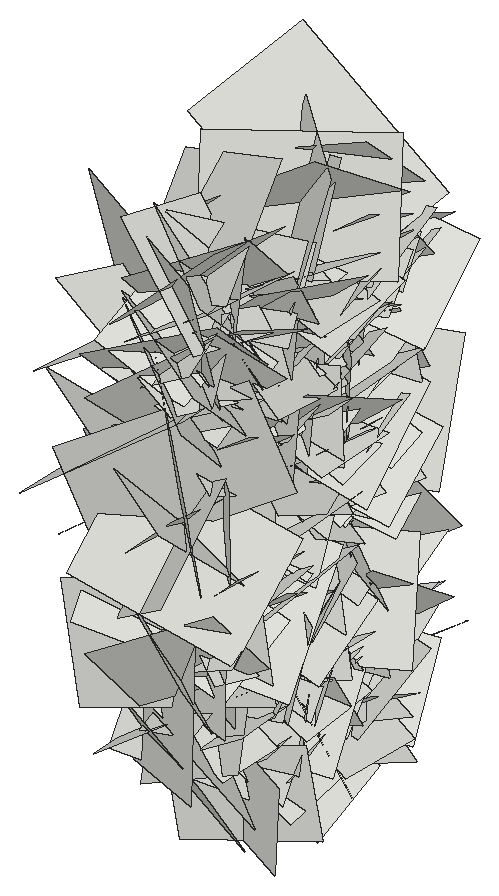
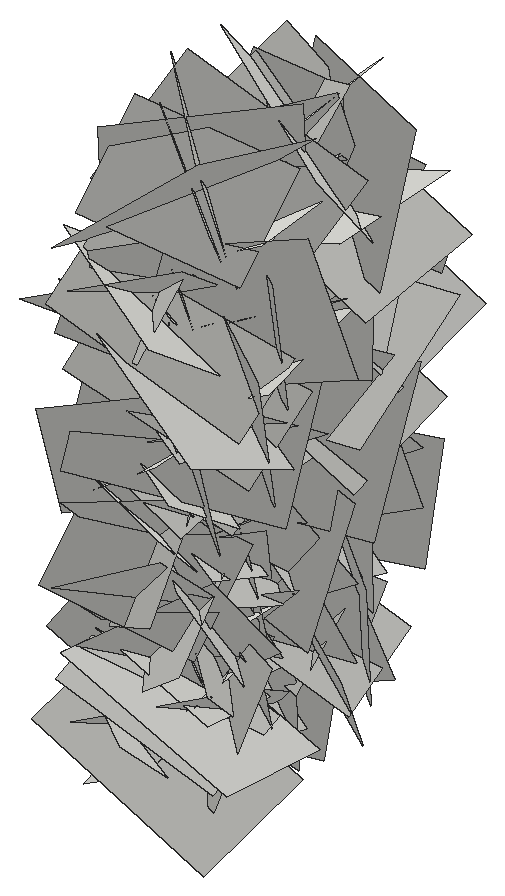
# SketchUp Ruby script. Lengths in inches.
U = 1.inch
M = Sketchup.active_model
def pt(a) = Geom::Point3d.new(a.map { |v| v * U })
def face(e, loops, mat)
  f = e.add_face(loops[0].map { |a| pt(a) })
  loops[1..].each { |l| e.add_face(l.map { |a| pt(a) }).erase! }
  f.material = f.back_material = mat if mat
  f
end
# faces: each face lists its corners as indices into pts; further lists are holes
def faces(e, pts, list, mat = nil) = list.each { |f| face(e, (f[0].is_a?(Array) ? f : [f]).map { |l| l.map { |i| pts[i] } }, mat) }
# xy, xz, yz: faces in a plane at the given z, y or x. An outline is a flat list of corners, or four numbers for a rectangle; further outlines are holes
def ring(l) = l.size == 4 ? [[l[0], l[1]], [l[2], l[1]], [l[2], l[3]], [l[0], l[3]]] : l.each_slice(2).to_a
def flat(e, list, mat, &to3) = list.each { |f| face(e, (f[0].is_a?(Array) ? f : [f]).map { |l| ring(l).map { |u, v| to3.(u, v) } }, mat) }
def xy(e, z, list, mat = nil) = flat(e, list, mat) { |x, y| [x, y, z] }
def xz(e, y, list, mat = nil) = flat(e, list, mat) { |x, z| [x, y, z] }
def yz(e, x, list, mat = nil) = flat(e, list, mat) { |y, z| [x, y, z] }
def lines(e, pts, list) = list.each { |a, b| e.add_line(pt(pts[a]), pt(pts[b])) }
# prism: a flat outline (further loops are holes) pulled along v
def prism(e, loops, v, mat = nil)
  f = face(e, loops, mat); d = Geom::Vector3d.new(v.map { |x| x * U })
  f.pushpull(f.normal.samedirection?(d) ? d.length : -d.length)
end
def box(e, o, s, mat = nil) = prism(e, [[o, [o[0] + s[0], o[1], o[2]], [o[0] + s[0], o[1] + s[1], o[2]], [o[0], o[1] + s[1], o[2]]]], [0, 0, s[2]], mat)
def at(x, y, z, deg = 0) = Geom::Transformation.translation(pt([x, y, z])) * Geom::Transformation.rotation(ORIGIN, Z_AXIS, deg.degrees)
def axes(o, x, y, z) = Geom::Transformation.new([*x, 0, *y, 0, *z, 0, *pt(o).to_a, 1])
def part(name) = M.definitions.add(name)
# library, detail: a bought-in or finely detailed component or shape, given as its bounding box
def library(name, o, s) = part(name).tap { |d| box(d.entities, o, s) }
def detail(e, o, s) = box(e.add_group.entities, o, s)
def put(e, d, t, mat = nil) = e.add_instance(d, t).tap { |i| i.material = mat if mat }
def group(e, t, mat = nil) = e.add_group.tap { |g| g.transformation = t; g.material = mat if mat }.entities
root = M.entities
c1 = part("Component\#6")
p = [[0.01,0,0],[0,3.24,4.54],[4.32,3.24,4.54],[4.33,0,0]]
faces(c1.entities,p,[[0,1,2,3]])
put(root,c1,axes([18.5,202.95,19.72],[-0.19445,-0.3512,-1.29554],[-0.25274,-1.27827,0.38028],[-1.40021,0.2795,0.11127]))
put(root,c1,axes([18.5,194.4,9.86],[-0.11876,-1.04596,0.91618],[-0.1474,0.92297,1.03671],[-1.46651,-0.00807,-0.1784]))
put(root,c1,axes([18.5,199.09,4.9],[-0.11121,1.25407,0.182],[-0.25083,0.16003,-1.23904],[-1.31962,-0.1361,0.22018]))
put(root,c1,axes([18.5,192.59,17.15],[-0.08597,-0.32374,1.28455],[-0.18245,1.27862,0.31138],[-1.3923,-0.14756,-0.12012]))
put(root,c1,axes([18.5,193.34,3.5],[-0.3285,0.68164,0.95344],[-0.04901,0.97833,-0.71446],[-1.2414,-0.219,-0.22409]))
put(root,c1,axes([18.5,197.84,15.77],[-0.08558,0.66637,-1.22765],[-0.01617,-1.23004,-0.66667],[-1.48057,-0.02508,0.07824]))
put(root,c1,axes([18.5,196.95,13.22],[-0.12152,0.35472,1.26895],[-0.01769,1.27325,-0.35743],[-1.39654,-0.047,-0.10589]))
put(root,c1,axes([18.5,198.6875,16.83],[-0.02201,1.26014,0.56955],[-0.0456,0.56875,-1.25994],[-1.46513,-0.03663,0.03065]))
put(root,c1,axes([18.5,191.67,21.5],[-0.0579,1.33618,-0.15223],[-0.05318,-0.15428,-1.33612],[-1.42453,-0.04855,0.05606]))
put(root,c1,axes([18.5,196.26,4.8],[-0.10051,-0.43998,1.12809],[-0.21352,1.12151,0.42048],[-1.26562,-0.15427,-0.16053]))
put(root,c1,axes([18.5,201.79,17.38],[-0.19939,0.73728,-1.06028],[0.09629,-1.06126,-0.75408],[-1.36551,-0.18249,0.10164]))
put(root,c1,axes([18.5,195.52,16.87],[-0.17814,-1.09516,0.21581],[-0.19304,0.24222,1.08736],[-1.16734,0.12707,-0.21275]))
put(root,c1,axes([18.5,190.86,3.39],[-0.21383,0.32739,1.20741],[0.09698,1.22359,-0.31649],[-1.32251,0.03679,-0.21843]))
put(root,c1,axes([18.5,190.45,18.05],[-0.16537,1.24759,-0.14593],[0.05265,-0.14081,-1.25691],[-1.33042,-0.16065,-0.0316]))
put(root,c1,axes([18.5,200.21,21.54],[-0.14018,1.21556,-0.55877],[0.14242,-0.54659,-1.22085],[-1.41094,-0.17594,-0.06772]))
put(root,c1,axes([18.5,192.73,15.73],[-0.12897,1.2724,-0.23633],[0.08155,-0.22984,-1.27707],[-1.36939,-0.13352,-0.05379]))
put(root,c1,axes([18.5,200.25,4.79],[-0.06637,1.27776,-0.24675],[0.01199,-0.2465,-1.2793],[-1.3794,-0.06362,0.00075]))
put(root,c1,axes([18.5,199.38,-0.0625],[-0.15183,-0.50198,1.07326],[-0.00307,1.08122,0.50532],[-1.25594,0.05804,-0.13098]))
put(root,c1,axes([18.5,192.7,21.39],[-0.08893,0.79245,0.9015],[-0.06254,0.89988,-0.79652],[-1.27076,-0.09974,-0.02389]))
put(root,c1,axes([18.5,194.09,6.34],[-0.25898,1.07168,-0.21064],[0.01285,-0.21318,-1.09862],[-1.15764,-0.24212,0.03493]))
put(root,c1,axes([18.5,200.7,5.85],[-0.20906,1.0682,-0.14016],[-0.07965,-0.15578,-1.08152],[-1.13921,-0.18514,0.10133]))
put(root,c1,axes([18.5,198.85,12.57],[-0.15345,0.48368,1.12599],[0.09378,1.13498,-0.47617],[-1.29562,0.02486,-0.16783]))
put(root,c1,axes([18.5,195.93,15.54],[-0.04965,0.25406,1.2028],[-0.02984,1.20314,-0.25523],[-1.30276,-0.03724,-0.03999]))
put(root,c1,axes([18.5,204.42,20.53],[-0.1154,-1.25003,-0.28156],[0.14973,-0.29256,1.24425],[-1.34995,0.07441,0.16208]))
put(root,c1,axes([18.5,199.56,18.73],[-0.07364,1.07871,-0.62029],[0.05176,-0.61841,-1.08091],[-1.31797,-0.08456,-0.00779]))
put(root,c1,axes([18.5,203.04,12.11],[-0.14841,-0.94408,-0.5752],[-0.05434,-0.57362,0.95398],[-1.17058,0.14632,0.02864]))
put(root,c1,axes([18.5,200.375,7.61],[-0.26418,-0.51362,-0.84712],[-0.05211,-0.86603,0.53955],[-1.04881,0.1724,0.18657]))
put(root,c1,axes([18.5,197.84,4.84],[-0.11369,-0.36766,-0.96616],[-0.19069,-0.94989,0.38144],[-1.07906,0.2066,0.03439]))
put(root,c1,axes([18.5,197.86,18.23],[-0.19608,0.2602,-1.0463],[0.01915,-1.06069,-0.26697],[-1.14269,-0.06243,0.17507]))
put(root,c1,axes([18.5,202.25,12.93],[0.19135,-1.27912,0.12446],[-0.2118,0.09622,1.27869],[-1.34571,-0.19703,-0.18355]))
put(root,c1,axes([18.5,198.375,11.05],[0.00636,-0.47599,-1.14741],[0.03555,-1.14695,0.47597],[-1.31628,-0.03327,0.00731]))
put(root,c1,axes([18.5,200.2,14.91],[-0.20407,-0.96139,-0.18597],[-0.07393,-0.17559,0.97991],[-1.03533,0.20204,-0.03331]))
put(root,c1,axes([18.5,196.53,2.03],[-0.14871,0.38131,0.94323],[-0.09041,0.94439,-0.39446],[-1.07463,-0.13222,-0.09734]))
put(root,c1,axes([18.5,192.66,5.0625],[-0.03803,0.06475,1.02957],[-0.25075,1.00223,-0.07127],[-1.06436,-0.23842,-0.02]))
put(root,c1,axes([18.5,199.09,16.39],[-0.13116,-1.14374,0.05938],[0.13174,0.04596,1.1443],[-1.20683,0.12933,0.11846]))
put(root,c1,axes([18.5,200.08,24.34],[-0.03463,0.75517,-0.67877],[-0.20748,-0.67107,-0.73718],[-1.05612,0.10708,0.16708]))
put(root,c1,axes([14.53,199.42,15.6],[-0.03605,-0.49998,-0.38134],[-0.14474,-0.36691,0.49324],[0.65063,-0.10932,0.0886]))
put(root,c1,axes([14.53,199.74,12.37],[-0.13977,-0.41949,-0.41774],[0.0557,-0.43458,0.41982],[0.62506,-0.05508,-0.13082]))
put(root,c1,axes([18.5,197.36,24.8],[0.09794,1.0389,-0.68546],[0.01654,-0.68826,-1.04104],[-1.31923,0.0685,-0.06394]))
put(root,c1,axes([18.5,194.35,10.5],[0.1187,0.07765,-1.12146],[-0.14385,-1.11784,-0.09095],[-1.18288,0.14373,-0.10148]))
put(root,c1,axes([18.5,194.25,1.05],[-0.1707,-0.55728,0.79671],[0.04122,0.80323,0.5697],[-1.02978,0.12452,-0.10926]))
put(root,c1,axes([18.5,205.24,14.9],[0.1168,-0.46047,-1.13614],[0.0362,-1.13913,0.465],[-1.29896,-0.07315,-0.0892]))
put(root,c1,axes([18.5,200.51,5.45],[0.07717,-0.59417,-0.91785],[-0.09928,-0.91989,0.58806],[-1.15472,0.03938,-0.1119]))
put(root,c1,axes([14.53,194.11,10.49],[-0.01019,-0.66626,0.06574],[-0.1187,0.06642,0.65679],[0.69967,0.00157,0.11238]))
put(root,c1,axes([18.5,202.1,18.26],[0.1919,-1.13475,-0.09678],[-0.16378,-0.12156,1.13628],[-1.19604,-0.16542,-0.17113]))
put(root,c1,axes([18.5,198.84,9.75],[0.24721,-0.9594,-0.88495],[0.06038,-0.89063,0.98057],[-1.38221,-0.2105,-0.11544]))
put(root,c1,axes([18.5,198.93,5.125],[-0.08676,0.85287,0.14934],[-0.16568,0.13299,-0.84515],[-0.90272,-0.10637,0.14076]))
put(root,c1,axes([18.5,203.91,5.3125],[-0.18463,-0.58129,-0.78091],[0.13848,-0.80009,0.56643],[-1.02258,-0.00339,0.2177]))
put(root,c1,axes([18.5,195.28,4.79],[-0.03702,0.87634,0.85063],[0.28559,0.83554,-0.84973],[-1.26267,0.16329,-0.21713]))
put(root,c1,axes([18.5,193.71,0.46],[-0.00413,-0.52236,0.7551],[-0.18121,0.74232,0.51263],[-0.95624,-0.13842,-0.10041]))
put(root,c1,axes([18.5,192.44,8.79],[0.05887,1.04295,0.25043],[-0.00297,0.2509,-1.04431],[-1.13694,0.05335,0.0157]))
put(root,c1,axes([14.53,196.1,5.28],[-0.08762,-0.56519,-0.39893],[0.0287,-0.4041,0.56691],[0.73275,-0.05175,-0.06991]))
put(root,c1,axes([14.53,199.53,17.66],[-0.07108,0.22718,0.77768],[-0.14032,0.76678,-0.23541],[0.84726,0.14605,0.02626]))
put(root,c1,axes([14.53,201.03,8.02],[-0.03451,-0.61291,-0.20918],[0.0475,-0.21108,0.61149],[0.68484,-0.01625,-0.05296]))
put(root,c1,axes([14.53,198.53,13.8],[-0.10676,-0.41647,0.70694],[-0.09382,0.7136,0.40779],[0.86465,0.02601,0.13154]))
put(root,c1,axes([18.5,196.19,13.89],[0.03711,0.95345,-0.08325],[-0.1071,-0.07916,-0.94908],[-1.00884,0.04348,0.09769]))
put(root,c1,axes([18.5,197.24,20.32],[-0.11105,0.4932,0.81979],[0.10012,0.82599,-0.48487],[-1.00916,0.02768,-0.13831]))
put(root,c1,axes([14.53,202.56,19.21],[0.06396,-0.26998,-0.58675],[-0.04641,-0.58965,0.26682],[0.68306,-0.01478,0.07307]))
put(root,c1,axes([14.53,199.64,2.06],[-0.21894,0.61345,0.59822],[0.01858,0.61825,-0.62794],[0.90807,0.13525,0.15708]))
put(root,c1,axes([18.5,196.07,8.125],[-0.08332,-0.69698,-0.457],[-0.10667,-0.44773,0.70016],[-0.87699,0.12068,-0.04174]))
put(root,c1,axes([14.53,190.79,19.57],[0.04866,0.55121,0.30162],[0.00575,0.30207,-0.55285],[0.66601,-0.04288,-0.01726]))
put(root,c1,axes([14.53,195.85,11.01],[-0.15114,0.73817,0.19544],[0.07767,0.21113,-0.74396],[0.80568,0.11812,0.10838]))
put(root,c1,axes([18.5,202.76,13.17],[0.11284,-1.03894,-0.17524],[-0.03066,-0.17895,1.04335],[-1.11641,-0.1001,-0.04636]))
put(root,c1,axes([18.5,189.31,11.46],[-0.01967,0.80876,0.77653],[0.21901,0.76581,-0.79265],[-1.16812,0.12996,-0.16169]))
put(root,c1,axes([14.53,193.57,4.75],[0.0218,0.6351,0.02763],[0.03876,0.02642,-0.63443],[0.67273,-0.0221,0.03566]))
put(root,c1,axes([18.5,199.68,18.17],[0.10811,0.81171,0.57509],[-0.11351,0.5837,-0.80488],[-1.04835,0.0205,0.14645]))
put(root,c1,axes([14.53,202.9,8.46],[-0.28421,-0.45126,-0.90988],[-0.10984,-0.92399,0.48879],[1.07096,-0.21452,-0.19133]))
put(root,c1,axes([14.53,193.91,15.9375],[0.03263,0.61645,-0.26034],[-0.02336,-0.25954,-0.61716],[0.70894,-0.03692,-0.00835]))
put(root,c1,axes([14.53,192.26,20.51],[-0.14395,0.6641,-0.62024],[-0.10915,-0.63433,-0.65665],[0.95701,0.02754,-0.16819]))
put(root,c1,axes([14.53,199.23,1.1],[-0.00098,-0.71414,-0.15761],[-0.04174,-0.15733,0.71311],[0.77408,-0.00939,0.03826]))
put(root,c1,axes([14.53,196.5625,6.92],[0.07674,-0.09799,-0.6482],[-0.03176,-0.65195,0.09521],[0.69417,-0.019,0.07601]))
put(root,c1,axes([14.53,198.91,12.75],[-0.15355,-0.10183,1.00426],[-0.21738,0.99636,0.07145],[1.04766,0.19182,0.16201]))
put(root,c1,axes([14.53,195.68,15.75],[0.06715,-0.51242,0.33521],[0.05381,0.34023,0.51051],[0.64683,0.02489,-0.07727]))
put(root,c1,axes([14.53,200.4375,8.06],[-0.17377,0.75884,-0.49804],[-0.05898,-0.51355,-0.76415],[0.96033,0.10576,-0.13705]))
put(root,c1,axes([14.53,199.6875,17.84],[0.07891,0.44569,0.39814],[0.07493,0.39183,-0.45185],[0.62903,-0.10259,0.00388]))
put(root,c1,axes([14.53,200.03,9.27],[-0.00412,-0.60297,0.30435],[0.07057,0.30253,0.60022],[0.71247,-0.03345,-0.05769]))
put(root,c1,axes([14.53,192.95,10.8],[0.02962,0.02518,0.78508],[-0.12702,0.77652,-0.02064],[0.82287,0.11896,-0.03145]))
put(root,c1,axes([18.5,199.37,10.67],[0.09558,-1.01864,0.46326],[0.13943,0.47118,1.01047],[-1.17795,-0.02688,0.1572]))
put(root,c1,axes([14.53,198.38,4.95],[-0.02223,0.32868,-0.55446],[0.17267,-0.53404,-0.32274],[0.66105,0.15055,0.06565]))
put(root,c1,axes([14.53,192.04,10.01],[-0.12172,0.5206,-0.6372],[0.01939,-0.6416,-0.52749],[0.87198,0.08694,-0.07722]))
put(root,c1,axes([14.53,202.51,19.98],[0.06792,0.48446,-0.5602],[-0.10116,-0.55221,-0.48846],[0.77852,-0.11402,-0.01459]))
put(root,c1,axes([18.5,195.86,16.68],[-0.06531,-0.43873,0.684],[-0.07025,0.68639,0.43429],[-0.8585,-0.02279,-0.08757]))
put(root,c1,axes([14.53,202.74,-0.14],[0.03158,-0.64507,0.25861],[0.01592,0.25938,0.64528],[0.73651,0.02205,-0.02503]))
put(root,c1,axes([18.5,192.22,20.81],[-0.00161,0.62306,-0.59539],[-0.0785,-0.59329,-0.62067],[-0.91013,0.05007,0.05459]))
put(root,c1,axes([14.53,197.35,3.52],[0.03443,0.41092,0.66217],[-0.08038,0.66126,-0.40665],[0.82215,0.04744,-0.06748]))
put(root,c1,axes([14.53,195.99,4.23],[-0.18601,0.0566,0.88651],[0.05201,0.90288,-0.04793],[0.94017,-0.03875,0.17804]))
put(root,c1,axes([18.5,198.67,11.97],[0.07539,0.76068,0.50866],[-0.0723,0.51318,-0.75791],[-0.96729,0.02092,0.0963]))
put(root,c1,axes([14.53,195.9375,9.16],[0.07841,0.69576,-0.29748],[-0.09095,-0.28926,-0.69787],[0.79692,-0.10147,-0.05038]))
put(root,c1,axes([18.5,195.4375,18.11],[-0.16874,-0.51977,-0.57708],[0.05885,-0.59519,0.52076],[-0.82114,0.06415,0.15591]))
put(root,c1,axes([18.5,196.17,12.88],[0.06274,0.02618,0.84664],[-0.15393,0.83645,-0.01571],[-0.88457,-0.1437,0.06278]))
put(root,c1,axes([18.5,193.46,10.77],[-0.10152,0.90556,-0.18731],[0.17799,-0.16815,-0.89879],[-0.96391,-0.12642,-0.14624]))
put(root,c1,axes([14.53,200.82,0.59],[0.02153,-0.73416,-0.35765],[-0.0933,-0.35764,0.72915],[0.8606,-0.02041,0.08799]))
put(root,c1,axes([18.5,195.73,16.63],[0.01219,-0.78698,0.32297],[-0.05977,0.32158,0.78561],[-0.89973,-0.03203,-0.04781]))
put(root,c1,axes([18.5,196.375,20.79],[0.12547,0.87042,-0.10702],[-0.18806,-0.08199,-0.86307],[-0.91037,0.1369,0.16354]))
put(root,c1,axes([18.5,200.05,13.66],[-0.07814,0.81604,-0.08962],[0.02759,-0.08761,-0.81916],[-0.86976,-0.0761,-0.01794]))
put(root,c1,axes([18.5,198.3125,4.47],[0.08144,0.93817,-0.09306],[0.01009,-0.09413,-0.94116],[-0.99929,0.07551,-0.01709]))
put(root,c1,axes([18.5,200.41,3.58],[0.05776,-0.87144,-0.04483],[-0.06577,-0.04867,0.87073],[-0.92261,-0.05109,-0.06488]))
put(root,c1,axes([18.5,195.95,14.86],[0.17446,0.9838,0.62037],[0.19333,0.59697,-0.99508],[-1.2176,0.23574,-0.06911]))
put(root,c1,axes([18.5,204.41,7.91],[-0.10208,-0.52254,-0.48763],[-0.08086,-0.48171,0.53127],[-0.75328,0.12252,0.00905]))
put(root,c1,axes([18.5,194.43,21.03],[0.18864,1.08922,-0.2367],[0.12278,-0.25647,-1.09312],[-1.17512,0.14806,-0.15221]))
put(root,c1,axes([14.53,200.69,6.875],[-0.16125,-0.91938,-0.30199],[-0.04119,-0.29965,0.93182],[1.02494,-0.15668,-0.01006]))
put(root,c1,axes([18.5,193.09,19.46],[-0.07295,0.25641,0.83596],[0.12348,0.83376,-0.24615],[-0.9186,0.09171,-0.09948]))
put(root,c1,axes([18.5,196.25,20.97],[-0.03433,0.46285,-0.75346],[0.09275,-0.74858,-0.46362],[-0.93272,-0.09148,-0.01837]))
put(root,c1,axes([14.53,193.9,23.36],[0.05376,0.55183,-0.55937],[-0.04326,-0.55793,-0.55411],[0.83178,-0.06469,0.00734]))
put(root,c1,axes([18.5,193.92,18.08],[0.13809,0.41624,-1.10581],[0.27382,-1.09563,-0.38198],[-1.22215,-0.19844,-0.21052]))
put(root,c1,axes([18.5,202.38,16.09],[0.07402,-0.92988,-0.45649],[0.17154,-0.44211,0.92536],[-1.08456,-0.13339,0.1152]))
put(root,c1,axes([14.53,201.99,11.3125],[-0.07595,0.62186,-0.76254],[-0.14567,-0.76339,-0.60964],[1.03278,-0.06194,-0.14206]))
put(root,c1,axes([14.53,202.11,15.27],[0.00741,-0.76642,-0.19435],[0.02033,-0.19414,0.76626],[0.83787,0.01149,-0.01688]))
put(root,c1,axes([18.5,195.27,-1.16],[0.10176,-0.07093,0.82892],[-0.16666,0.81783,0.08819],[-0.86597,-0.16573,0.08043]))
put(root,c1,axes([18.5,196.11,19.5625],[0.1708,0.27531,1.11719],[0.21419,1.10379,-0.30115],[-1.2007,0.23607,0.1052]))
put(root,c1,axes([14.53,200.46,4.14],[0.03987,0.66432,-0.22968],[0.12809,-0.2327,-0.65325],[0.73398,0.00452,0.12648]))
put(root,c1,axes([18.5,200.85,9.74],[-0.02518,0.49854,0.49521],[-0.19267,0.47427,-0.48618],[-0.7195,-0.14445,0.11286]))
put(root,c1,axes([14.53,192.1875,23.6],[0.04344,0.89705,-0.17333],[-0.1764,-0.16328,-0.88435],[0.95226,-0.07116,-0.15591]))
put(root,c1,axes([18.5,192.1875,23.6],[-0.04344,0.89705,-0.17333],[0.1764,-0.16328,-0.88435],[-0.95226,-0.07116,-0.15591]))
put(root,c1,axes([14.53,200.85,9.74],[0.02518,0.49854,0.49521],[0.19267,0.47427,-0.48618],[0.7195,-0.14445,0.11286]))
put(root,c1,axes([18.5,200.46,4.14],[-0.03987,0.66432,-0.22968],[-0.12809,-0.2327,-0.65325],[-0.73398,0.00452,0.12648]))
put(root,c1,axes([14.53,196.11,19.5625],[-0.1708,0.27531,1.11719],[-0.21419,1.10379,-0.30115],[1.2007,0.23607,0.1052]))
put(root,c1,axes([14.53,195.27,-1.16],[-0.10176,-0.07093,0.82892],[0.16666,0.81783,0.08819],[0.86597,-0.16573,0.08043]))
put(root,c1,axes([18.5,202.11,15.27],[-0.00741,-0.76642,-0.19435],[-0.02033,-0.19414,0.76626],[-0.83787,0.01149,-0.01688]))
put(root,c1,axes([18.5,201.99,11.3125],[0.07595,0.62186,-0.76254],[0.14567,-0.76339,-0.60964],[-1.03278,-0.06194,-0.14206]))
put(root,c1,axes([14.53,202.38,16.09],[-0.07402,-0.92988,-0.45649],[-0.17154,-0.44211,0.92536],[1.08456,-0.13339,0.1152]))
put(root,c1,axes([14.53,193.92,18.08],[-0.13809,0.41624,-1.10581],[-0.27382,-1.09563,-0.38198],[1.22215,-0.19844,-0.21052]))
put(root,c1,axes([18.5,193.9,23.36],[-0.05376,0.55183,-0.55937],[0.04326,-0.55793,-0.55411],[-0.83178,-0.06469,0.00734]))
put(root,c1,axes([14.53,196.25,20.97],[0.03433,0.46285,-0.75346],[-0.09275,-0.74858,-0.46362],[0.93272,-0.09148,-0.01837]))
put(root,c1,axes([14.53,193.09,19.46],[0.07295,0.25641,0.83596],[-0.12348,0.83376,-0.24615],[0.9186,0.09171,-0.09948]))
put(root,c1,axes([18.5,200.69,6.875],[0.16125,-0.91938,-0.30199],[0.04119,-0.29965,0.93182],[-1.02494,-0.15668,-0.01006]))
put(root,c1,axes([14.53,194.43,21.03],[-0.18864,1.08922,-0.2367],[-0.12278,-0.25647,-1.09312],[1.17512,0.14806,-0.15221]))
put(root,c1,axes([14.53,195.95,14.86],[-0.17446,0.9838,0.62037],[-0.19333,0.59697,-0.99508],[1.2176,0.23574,-0.06911]))
put(root,c1,axes([14.53,200.41,3.58],[-0.05776,-0.87144,-0.04483],[0.06577,-0.04867,0.87073],[0.92261,-0.05109,-0.06488]))
put(root,c1,axes([14.53,198.3125,4.47],[-0.08144,0.93817,-0.09306],[-0.01009,-0.09413,-0.94116],[0.99929,0.07551,-0.01709]))
put(root,c1,axes([14.53,200.05,13.66],[0.07814,0.81604,-0.08962],[-0.02759,-0.08761,-0.81916],[0.86976,-0.0761,-0.01794]))
put(root,c1,axes([14.53,196.375,20.79],[-0.12547,0.87042,-0.10702],[0.18806,-0.08199,-0.86307],[0.91037,0.1369,0.16354]))
put(root,c1,axes([14.53,195.73,16.63],[-0.01219,-0.78698,0.32297],[0.05977,0.32158,0.78561],[0.89973,-0.03203,-0.04781]))
put(root,c1,axes([18.5,200.82,0.59],[-0.02153,-0.73416,-0.35765],[0.0933,-0.35764,0.72915],[-0.8606,-0.02041,0.08799]))
put(root,c1,axes([14.53,193.46,10.77],[0.10152,0.90556,-0.18731],[-0.17799,-0.16815,-0.89879],[0.96391,-0.12642,-0.14624]))
put(root,c1,axes([14.53,196.17,12.88],[-0.06274,0.02618,0.84664],[0.15393,0.83645,-0.01571],[0.88457,-0.1437,0.06278]))
put(root,c1,axes([14.53,195.4375,18.11],[0.16874,-0.51977,-0.57708],[-0.05885,-0.59519,0.52076],[0.82114,0.06415,0.15591]))
put(root,c1,axes([18.5,195.9375,9.16],[-0.07841,0.69576,-0.29748],[0.09095,-0.28926,-0.69787],[-0.79692,-0.10147,-0.05038]))
put(root,c1,axes([14.53,198.67,11.97],[-0.07539,0.76068,0.50866],[0.0723,0.51318,-0.75791],[0.96729,0.02092,0.0963]))
put(root,c1,axes([18.5,195.99,4.23],[0.18601,0.0566,0.88651],[-0.05201,0.90288,-0.04793],[-0.94017,-0.03875,0.17804]))
put(root,c1,axes([18.5,197.35,3.52],[-0.03443,0.41092,0.66217],[0.08038,0.66126,-0.40665],[-0.82215,0.04744,-0.06748]))
put(root,c1,axes([14.53,192.22,20.81],[0.00161,0.62306,-0.59539],[0.0785,-0.59329,-0.62067],[0.91013,0.05007,0.05459]))
put(root,c1,axes([18.5,202.74,-0.14],[-0.03158,-0.64507,0.25861],[-0.01592,0.25938,0.64528],[-0.73651,0.02205,-0.02503]))
put(root,c1,axes([14.53,195.86,16.68],[0.06531,-0.43873,0.684],[0.07025,0.68639,0.43429],[0.8585,-0.02279,-0.08757]))
put(root,c1,axes([18.5,202.51,19.98],[-0.06792,0.48446,-0.5602],[0.10116,-0.55221,-0.48846],[-0.77852,-0.11402,-0.01459]))
put(root,c1,axes([18.5,192.04,10.01],[0.12172,0.5206,-0.6372],[-0.01939,-0.6416,-0.52749],[-0.87198,0.08694,-0.07722]))
put(root,c1,axes([18.5,198.38,4.95],[0.02223,0.32868,-0.55446],[-0.17267,-0.53404,-0.32274],[-0.66105,0.15055,0.06565]))
put(root,c1,axes([14.53,199.37,10.67],[-0.09558,-1.01864,0.46326],[-0.13943,0.47118,1.01047],[1.17795,-0.02688,0.1572]))
put(root,c1,axes([18.5,192.95,10.8],[-0.02962,0.02518,0.78508],[0.12702,0.77652,-0.02064],[-0.82287,0.11896,-0.03145]))
put(root,c1,axes([18.5,200.03,9.27],[0.00412,-0.60297,0.30435],[-0.07057,0.30253,0.60022],[-0.71247,-0.03345,-0.05769]))
put(root,c1,axes([18.5,199.6875,17.84],[-0.07891,0.44569,0.39814],[-0.07493,0.39183,-0.45185],[-0.62903,-0.10259,0.00388]))
put(root,c1,axes([18.5,200.4375,8.06],[0.17377,0.75884,-0.49804],[0.05898,-0.51355,-0.76415],[-0.96033,0.10576,-0.13705]))
put(root,c1,axes([18.5,195.68,15.75],[-0.06715,-0.51242,0.33521],[-0.05381,0.34023,0.51051],[-0.64683,0.02489,-0.07727]))
put(root,c1,axes([18.5,198.91,12.75],[0.15355,-0.10183,1.00426],[0.21738,0.99636,0.07145],[-1.04766,0.19182,0.16201]))
put(root,c1,axes([18.5,196.5625,6.92],[-0.07674,-0.09799,-0.6482],[0.03176,-0.65195,0.09521],[-0.69417,-0.019,0.07601]))
put(root,c1,axes([18.5,199.23,1.1],[0.00098,-0.71414,-0.15761],[0.04174,-0.15733,0.71311],[-0.77408,-0.00939,0.03826]))
put(root,c1,axes([18.5,192.26,20.51],[0.14395,0.6641,-0.62024],[0.10915,-0.63433,-0.65665],[-0.95701,0.02754,-0.16819]))
put(root,c1,axes([18.5,193.91,15.9375],[-0.03263,0.61645,-0.26034],[0.02336,-0.25954,-0.61716],[-0.70894,-0.03692,-0.00835]))
put(root,c1,axes([18.5,202.9,8.46],[0.28421,-0.45126,-0.90988],[0.10984,-0.92399,0.48879],[-1.07096,-0.21452,-0.19133]))
put(root,c1,axes([14.53,199.68,18.17],[-0.10811,0.81171,0.57509],[0.11351,0.5837,-0.80488],[1.04835,0.0205,0.14645]))
put(root,c1,axes([18.5,193.57,4.75],[-0.0218,0.6351,0.02763],[-0.03876,0.02642,-0.63443],[-0.67273,-0.0221,0.03566]))
put(root,c1,axes([14.53,189.31,11.46],[0.01967,0.80876,0.77653],[-0.21901,0.76581,-0.79265],[1.16812,0.12996,-0.16169]))
put(root,c1,axes([14.53,202.76,13.17],[-0.11284,-1.03894,-0.17524],[0.03066,-0.17895,1.04335],[1.11641,-0.1001,-0.04636]))
put(root,c1,axes([18.5,195.85,11.01],[0.15114,0.73817,0.19544],[-0.07767,0.21113,-0.74396],[-0.80568,0.11812,0.10838]))
put(root,c1,axes([18.5,190.79,19.57],[-0.04866,0.55121,0.30162],[-0.00575,0.30207,-0.55285],[-0.66601,-0.04288,-0.01726]))
put(root,c1,axes([14.53,196.07,8.125],[0.08332,-0.69698,-0.457],[0.10667,-0.44773,0.70016],[0.87699,0.12068,-0.04174]))
put(root,c1,axes([18.5,199.64,2.06],[0.21894,0.61345,0.59822],[-0.01858,0.61825,-0.62794],[-0.90807,0.13525,0.15708]))
put(root,c1,axes([18.5,202.56,19.21],[-0.06396,-0.26998,-0.58675],[0.04641,-0.58965,0.26682],[-0.68306,-0.01478,0.07307]))
